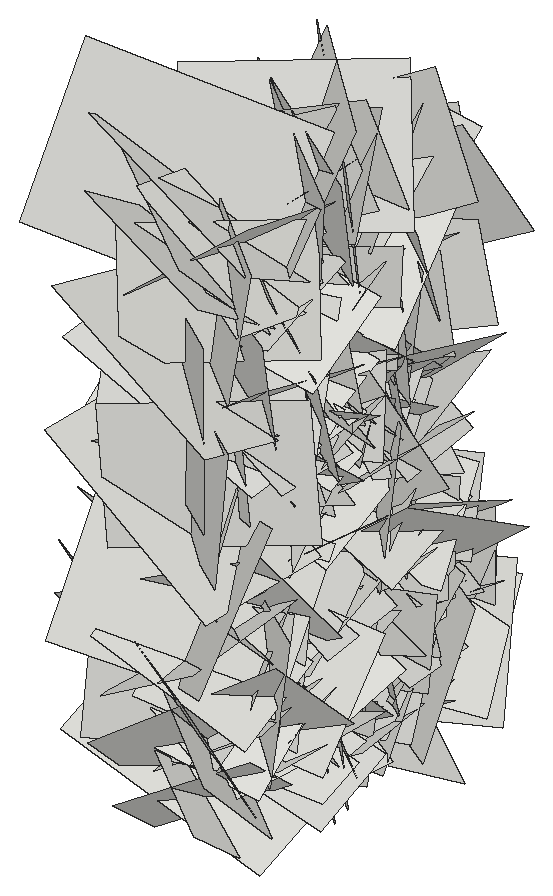
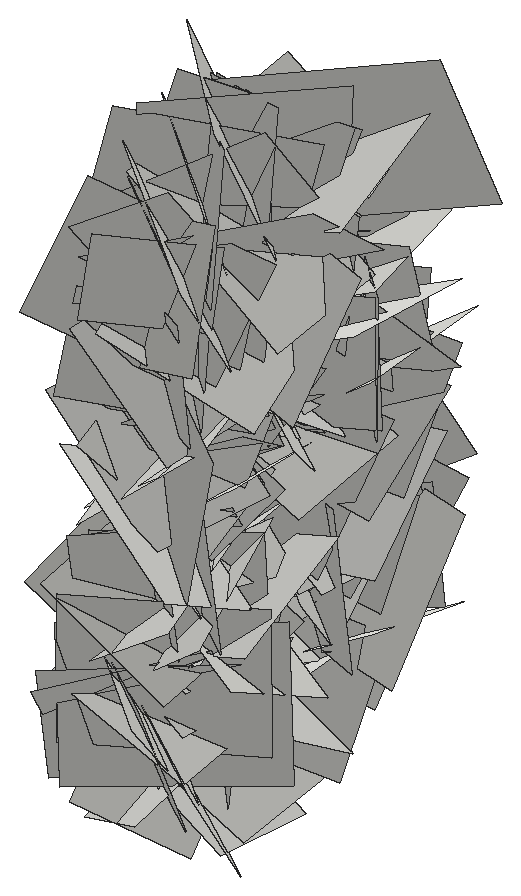
# SketchUp Ruby script. Lengths in inches.
U = 1.inch
M = Sketchup.active_model
def pt(a) = Geom::Point3d.new(a.map { |v| v * U })
def face(e, loops, mat)
  f = e.add_face(loops[0].map { |a| pt(a) })
  loops[1..].each { |l| e.add_face(l.map { |a| pt(a) }).erase! }
  f.material = f.back_material = mat if mat
  f
end
# faces: each face lists its corners as indices into pts; further lists are holes
def faces(e, pts, list, mat = nil) = list.each { |f| face(e, (f[0].is_a?(Array) ? f : [f]).map { |l| l.map { |i| pts[i] } }, mat) }
# xy, xz, yz: faces in a plane at the given z, y or x. An outline is a flat list of corners, or four numbers for a rectangle; further outlines are holes
def ring(l) = l.size == 4 ? [[l[0], l[1]], [l[2], l[1]], [l[2], l[3]], [l[0], l[3]]] : l.each_slice(2).to_a
def flat(e, list, mat, &to3) = list.each { |f| face(e, (f[0].is_a?(Array) ? f : [f]).map { |l| ring(l).map { |u, v| to3.(u, v) } }, mat) }
def xy(e, z, list, mat = nil) = flat(e, list, mat) { |x, y| [x, y, z] }
def xz(e, y, list, mat = nil) = flat(e, list, mat) { |x, z| [x, y, z] }
def yz(e, x, list, mat = nil) = flat(e, list, mat) { |y, z| [x, y, z] }
def lines(e, pts, list) = list.each { |a, b| e.add_line(pt(pts[a]), pt(pts[b])) }
# prism: a flat outline (further loops are holes) pulled along v
def prism(e, loops, v, mat = nil)
  f = face(e, loops, mat); d = Geom::Vector3d.new(v.map { |x| x * U })
  f.pushpull(f.normal.samedirection?(d) ? d.length : -d.length)
end
def box(e, o, s, mat = nil) = prism(e, [[o, [o[0] + s[0], o[1], o[2]], [o[0] + s[0], o[1] + s[1], o[2]], [o[0], o[1] + s[1], o[2]]]], [0, 0, s[2]], mat)
def at(x, y, z, deg = 0) = Geom::Transformation.translation(pt([x, y, z])) * Geom::Transformation.rotation(ORIGIN, Z_AXIS, deg.degrees)
def axes(o, x, y, z) = Geom::Transformation.new([*x, 0, *y, 0, *z, 0, *pt(o).to_a, 1])
def part(name) = M.definitions.add(name)
# library, detail: a bought-in or finely detailed component or shape, given as its bounding box
def library(name, o, s) = part(name).tap { |d| box(d.entities, o, s) }
def detail(e, o, s) = box(e.add_group.entities, o, s)
def put(e, d, t, mat = nil) = e.add_instance(d, t).tap { |i| i.material = mat if mat }
def group(e, t, mat = nil) = e.add_group.tap { |g| g.transformation = t; g.material = mat if mat }.entities
root = M.entities
c1 = part("Component\#6")
p = [[0.01,0,0],[0,3.24,4.54],[4.32,3.24,4.54],[4.33,0,0]]
faces(c1.entities,p,[[0,1,2,3]])
put(root,c1,axes([18.5,141.18,23.91],[-0.20239,-0.45291,-1.29893],[-0.24414,-1.28235,0.48098],[-1.43758,0.28153,0.10118]))
put(root,c1,axes([18.5,137.06,3.09],[-0.11239,-0.69918,1.17187],[-0.18512,1.17269,0.68387],[-1.43458,-0.09655,-0.18006]))
put(root,c1,axes([18.5,140.96,14.21],[-0.1647,-0.56811,1.02456],[-0.16232,1.03452,0.5504],[-1.23116,-0.0604,-0.20963]))
put(root,c1,axes([18.5,141.32,18.93],[0.00931,-1.12138,0.55372],[-0.26786,0.54072,1.09906],[-1.29833,-0.1196,-0.22278]))
put(root,c1,axes([18.5,142.16,14.375],[0.02255,-1.26636,-0.09652],[-0.2141,-0.09868,1.25016],[-1.3291,-0.00559,-0.20302]))
put(root,c1,axes([18.5,139.3125,6.46],[0.05297,-0.89114,0.82127],[-0.332,0.78454,0.87035],[-1.24093,-0.24794,-0.1978]))
put(root,c1,axes([18.5,148.13,7.79],[-0.13698,0.11741,-1.23467],[0.05668,-1.23967,-0.12348],[-1.31343,-0.06574,0.12344]))
put(root,c1,axes([18.5,134.59,13.6],[-0.14779,0.17555,1.29716],[0.16453,1.29751,-0.15892],[-1.37773,0.13612,-0.15813]))
put(root,c1,axes([18.5,141.11,14.91],[-0.10517,-0.78429,-0.79452],[-0.18451,-0.77703,0.78876],[-1.16892,0.19321,-0.05302]))
put(root,c1,axes([18.5,144.73,5.33],[-0.04426,-1.02294,0.56209],[-0.16257,0.56238,1.01208],[-1.2265,-0.03763,-0.15444]))
put(root,c1,axes([18.5,144.3,10.94],[-0.16969,-0.07735,1.18237],[0.06112,1.19119,0.08573],[-1.2545,0.0685,-0.15576]))
put(root,c1,axes([18.5,148.05,8.79],[-0.07068,0.0827,-1.14811],[-0.1221,-1.14474,-0.07576],[-1.21402,0.11031,0.07447]))
put(root,c1,axes([18.5,138.37,16.22],[-0.07456,0.76169,-0.90937],[-0.0504,-0.91204,-0.76025],[-1.25638,-0.00862,0.08446]))
put(root,c1,axes([18.5,141.48,7.17],[-0.20337,0.82379,-0.77749],[0.08888,-0.77608,-0.84298],[-1.19742,-0.19752,0.06948]))
put(root,c1,axes([18.5,139.44,14.86],[0.04621,-1.16691,0.31838],[-0.12643,0.31289,1.16311],[-1.27589,-0.07327,-0.10372]))
put(root,c1,axes([18.5,139.77,22.87],[-0.12093,1.26112,-0.05281],[0.18505,-0.03675,-1.25475],[-1.32509,-0.12022,-0.17041]))
put(root,c1,axes([18.5,146.96,20.2],[0.19126,-1.0536,-0.82739],[-0.10265,-0.84293,1.05228],[-1.41631,-0.08119,-0.188]))
put(root,c1,axes([18.5,137.94,15.45],[0.03401,0.89045,-0.73196],[-0.17038,-0.72163,-0.88493],[-1.2099,0.12665,0.10405]))
put(root,c1,axes([18.5,140.59,7.56],[0.03383,1.06332,0.50099],[-0.10932,0.50178,-1.05842],[-1.24115,-0.01522,0.10688]))
put(root,c1,axes([18.5,140.04,10.48],[0.03722,-1.27767,0.05021],[0.04996,0.05148,1.27723],[-1.35446,-0.03321,0.04849]))
put(root,c1,axes([18.5,143.08,17.68],[0.06532,-0.13436,-1.17102],[-0.13166,-1.16683,0.12734],[-1.24247,0.11658,-0.07506]))
put(root,c1,axes([18.5,141.75,2.91],[0.11729,-1.19784,-0.30033],[-0.11289,-0.30967,1.19584],[-1.30414,-0.08092,-0.13053]))
put(root,c1,axes([18.5,140.93,18.6875],[0.10901,-0.41314,-1.06231],[-0.28274,-1.04573,0.38087],[-1.17466,0.21337,-0.19026]))
put(root,c1,axes([18.5,137.64,18.89],[-0.26376,-0.64139,0.69016],[-0.02251,0.71746,0.65911],[-0.99845,0.15326,-0.19718]))
put(root,c1,axes([18.5,142.88,1.98],[-0.0351,0.64216,0.95117],[-0.00533,0.95147,-0.64254],[-1.21649,-0.02269,-0.02463]))
put(root,c1,axes([18.5,143.17,19.13],[-0.20193,0.9279,-0.28366],[-0.04691,-0.29708,-0.94209],[-1.02744,-0.16881,0.09877]))
put(root,c1,axes([18.5,137.21,11.6875],[0.11385,0.72886,-0.88593],[-0.14818,-0.87485,-0.7367],[-1.20699,0.17615,0.00688]))
put(root,c1,axes([14.53,137.29,3.46],[-0.14224,0.61257,0.15159],[0.04066,0.16261,-0.62315],[0.66768,0.1206,0.07024]))
put(root,c1,axes([18.5,138.49,4.97],[0.13436,1.04009,0.6085],[-0.04809,0.61554,-1.04268],[-1.27641,0.08629,0.10334]))
put(root,c1,axes([18.5,138.64,15.1],[0.05154,1.07135,-0.23626],[-0.10153,-0.23144,-1.06922],[-1.15847,0.06794,0.08319]))
put(root,c1,axes([18.5,142.72,8.07],[0.13823,0.05764,1.30603],[0.0986,1.30878,-0.06705],[-1.38223,0.09912,0.12583]))
put(root,c1,axes([14.53,142.82,6.12],[0.04161,-0.60559,-0.03198],[-0.13563,-0.03959,0.59276],[0.62835,0.03156,0.13006]))
put(root,c1,axes([18.5,143.54,11.83],[0.01207,0.98557,0.48784],[-0.03058,0.48797,-0.98515],[-1.16528,-0.0026,0.03091]))
put(root,c1,axes([18.5,141.07,4.77],[0.0925,1.07709,-0.24358],[-0.13853,-0.23255,-1.07513],[-1.16232,0.11343,0.10875]))
put(root,c1,axes([18.5,137.41,10.49],[-0.17918,0.96529,0.20208],[0.06958,0.21558,-0.97489],[-1.04307,-0.15144,-0.09975]))
put(root,c1,axes([18.5,139.52,8.83],[-0.01584,-0.12995,-1.07448],[-0.00128,-1.07458,0.12998],[-1.14724,0.003,0.01469]))
put(root,c1,axes([18.5,138.76,9.15],[-0.08107,-0.07376,-0.93469],[-0.12107,-0.93007,0.08274],[-0.98644,0.12021,0.06666]))
put(root,c1,axes([18.5,138.34,13.4],[-0.1901,0.66514,0.65147],[0.02496,0.66648,-0.67398],[-0.98658,-0.1113,-0.14258]))
put(root,c1,axes([18.5,141.92,3.18],[-0.02887,1.0089,0.10446],[-0.06921,0.10254,-1.00735],[-1.07292,-0.03376,0.06217]))
put(root,c1,axes([14.53,139.18,13.74],[-0.11062,-0.13563,-0.63299],[0.03095,-0.6415,0.13263],[0.6855,0.00708,-0.10814]))
put(root,c1,axes([18.5,137.89,18.97],[-0.02244,-0.79516,0.48934],[-0.22215,0.48102,0.77258],[-0.96443,-0.0923,-0.18934]))
put(root,c1,axes([18.5,137.63,3.85],[0.23328,-0.07655,1.22947],[-0.08564,1.24535,0.092],[-1.30295,-0.09556,0.21407]))
put(root,c1,axes([14.53,141.95,12.73],[-0.09992,0.55515,0.3498],[0.02862,0.35638,-0.5583],[0.69495,0.06514,0.07329]))
put(root,c1,axes([18.5,146.45,10.34],[-0.10559,0.05407,-0.92917],[-0.0532,-0.93343,-0.04894],[-0.98516,0.04461,0.10223]))
put(root,c1,axes([14.53,145.42,18.19],[-0.07853,-0.05807,0.70782],[-0.06912,0.70921,0.05136],[0.74963,0.05931,0.07889]))
put(root,c1,axes([14.53,145.36,10.15],[-0.14636,-0.64891,0.3527],[-0.01811,0.36152,0.65845],[0.78267,-0.11298,0.08119]))
put(root,c1,axes([14.53,142.6,14.22],[-0.18899,-0.6396,-0.42028],[0.00285,-0.43205,0.65638],[0.81124,-0.14749,-0.10022]))
put(root,c1,axes([14.53,139.8125,20.98],[0.02151,0.52563,-0.34386],[-0.05265,-0.34162,-0.52514],[0.66372,-0.04413,-0.03051]))
put(root,c1,axes([18.5,144.58,9.97],[-0.16827,0.58944,-0.69808],[0.0398,-0.70373,-0.60275],[-0.96765,-0.13145,0.0966]))
put(root,c1,axes([18.5,142.29,19.52],[-0.02505,0.60517,0.90894],[0.1077,0.90642,-0.60085],[-1.15246,0.07156,-0.07591]))
put(root,c1,axes([18.5,137.99,14.66],[0.08461,-0.27233,0.9902],[-0.1352,0.98287,0.28059],[-1.08015,-0.14435,0.04245]))
put(root,c1,axes([18.5,144.34,6.82],[0.01542,0.93301,-0.17325],[-0.14993,-0.1692,-0.92309],[-0.99466,0.03997,0.13646]))
put(root,c1,axes([18.5,141.25,1.55],[-0.11713,-0.0063,1.0149],[0.13715,1.01248,0.02037],[-1.06704,0.13083,-0.10878]))
put(root,c1,axes([18.5,142.2,15.72],[0.2001,0.61396,-1.10583],[0.10306,-1.12181,-0.60624],[-1.33676,0.00542,-0.21228]))
put(root,c1,axes([14.53,138.3,10.21],[-0.07821,-0.14386,0.79141],[-0.12147,0.78851,0.13265],[0.84394,0.10016,0.09244]))
put(root,c1,axes([14.53,147.58,14.43],[-0.15626,-0.88067,0.15465],[-0.14549,0.17716,0.87807],[0.93656,-0.11942,0.1622]))
put(root,c1,axes([14.53,139.99,14.29],[0.01199,-0.16574,0.68191],[-0.09091,0.67656,0.16586],[0.73829,0.086,0.00935]))
put(root,c1,axes([18.5,139.9,15.42],[-0.08068,-0.00169,-0.87701],[-0.08263,-0.87681,0.00845],[-0.92595,0.07839,0.07566]))
put(root,c1,axes([14.53,145.32,5.58],[0.01721,-0.24816,-0.73855],[-0.187,-0.7207,0.23828],[0.80443,-0.16223,0.07119]))
put(root,c1,axes([18.5,140.66,10.67],[0.05387,-0.70807,-1.02445],[0.25854,-0.99979,0.70312],[-1.29449,-0.22915,0.09779]))
put(root,c1,axes([18.5,141.11,17.69],[-0.01651,0.23078,-0.87547],[-0.12637,-0.8685,-0.22682],[-0.95135,0.11136,0.04532]))
put(root,c1,axes([14.53,138.56,10.4375],[-0.05239,0.37979,0.51244],[0.10197,0.51253,-0.37059],[0.66837,-0.04842,0.0967]))
put(root,c1,axes([18.5,149.05,6.52],[0.16475,-0.3536,-1.09271],[0.00842,-1.10231,0.35784],[-1.21738,-0.05548,-0.1454]))
put(root,c1,axes([18.5,142.09,4.39],[-0.13266,-0.06807,0.83796],[-0.05074,0.84639,0.06161],[-0.88972,-0.03812,-0.12846]))
put(root,c1,axes([18.5,136.25,6.15],[-0.02753,0.62765,0.83331],[0.11118,0.83092,-0.62258],[-1.10023,0.06826,-0.08377]))
put(root,c1,axes([14.53,141.82,12.65],[0.04235,0.31596,0.66399],[-0.14644,0.65635,-0.30401],[0.76557,0.10807,-0.09488]))
put(root,c1,axes([18.5,145.41,21.68],[-0.17174,-0.50133,-0.77339],[0.12403,-0.79008,0.48764],[-0.96905,-0.01227,0.19948]))
put(root,c1,axes([14.53,139.97,19.34],[-0.20036,-0.21311,0.82685],[-0.01235,0.84743,0.21575],[0.90502,-0.03562,0.186]))
put(root,c1,axes([18.5,135.11,11.54],[0.10699,0.00448,1.06975],[-0.01257,1.07444,-0.00338],[-1.13388,-0.01149,0.10098]))
put(root,c1,axes([14.53,141.75,2.2],[0.07408,-0.19814,0.56205],[0.01701,0.56632,0.19765],[0.63148,0.00798,-0.07126]))
put(root,c1,axes([18.5,137.79,2.1],[0.03475,-0.78477,0.75119],[0.11687,0.75006,0.77877],[-1.14558,0.05272,0.10224]))
put(root,c1,axes([14.53,139.2,5.38],[-0.02645,-0.5119,-0.36479],[0.13209,-0.36186,0.49927],[0.65307,0.05245,-0.11575]))
put(root,c1,axes([14.53,147.44,21.48],[0.11936,-0.32986,-0.48912],[-0.02265,-0.49991,0.33221],[0.62494,0.04489,0.10546]))
put(root,c1,axes([18.5,139.48,6.78],[-0.1397,0.74364,0.31774],[-0.04551,0.31504,-0.75514],[-0.85599,-0.13812,-0.01171]))
put(root,c1,axes([18.5,146.4375,4.35],[0.18242,-1.06895,0.55133],[0.10581,0.56772,1.06956],[-1.27052,-0.1062,0.16823]))
put(root,c1,axes([14.53,141.96,13.08],[0.07799,-0.57044,-0.33182],[-0.05167,-0.33766,0.56968],[0.69762,0.03877,0.07929]))
put(root,c1,axes([18.5,137.55,18.4],[0.05522,0.7917,0.38208],[-0.20111,0.38385,-0.76951],[-0.90986,-0.0368,0.19328]))
put(root,c1,axes([14.53,140.67,1.375],[0.09858,-0.02009,0.69473],[-0.09996,0.69407,0.03269],[0.72991,0.09776,-0.08935]))
put(root,c1,axes([14.53,143.63,3.63],[0.04495,-0.13338,0.65571],[0.00407,0.65706,0.13341],[0.70927,0.00468,-0.04233]))
put(root,c1,axes([14.53,139.35,17.19],[0.06054,-0.33637,0.61942],[-0.0607,0.61718,0.34043],[0.74468,0.07766,-0.02261]))
put(root,c1,axes([18.5,145.52,15.88],[0.20612,-0.51117,0.96001],[-0.04532,0.97089,0.52562],[-1.15198,-0.12966,0.1511]))
put(root,c1,axes([14.53,136.74,12.93],[0.11437,0.04247,0.59628],[0.02624,0.60507,-0.04758],[0.63311,-0.03275,-0.10574]))
put(root,c1,axes([14.53,142.73,15.75],[-0.26089,1.021,-0.12695],[-0.10549,-0.15355,-1.04195],[1.08548,0.23047,-0.13178]))
put(root,c1,axes([18.5,139.41,15.5],[-0.07329,-0.02436,0.98546],[0.16551,0.97513,0.03506],[-1.03171,0.15816,-0.06438]))
put(root,c1,axes([14.53,143.53,7.33],[-0.11895,-0.88372,0.009],[-0.0734,0.01784,0.88799],[0.93392,-0.11115,0.07094]))
put(root,c1,axes([18.5,142.07,24.73],[0.13514,0.30002,-0.93652],[-0.09595,-0.93677,-0.31242],[-1.03799,0.12565,-0.09305]))
put(root,c1,axes([14.53,138.58,20.36],[-0.30182,0.3301,1.08442],[-0.18064,1.09293,-0.37743],[1.1879,0.25007,0.21813]))
put(root,c1,axes([18.5,143.76,15.19],[-0.09057,0.86782,-0.29614],[0.1091,-0.28647,-0.86917],[-0.96584,-0.11373,-0.07041]))
put(root,c1,axes([18.5,139.77,3.95],[-0.11908,-0.78329,-0.0515],[-0.03618,-0.0471,0.79084],[-0.83129,0.11425,-0.02704]))
put(root,c1,axes([14.53,146.8125,4.55],[-0.17148,-0.83232,0.10491],[0.08015,0.09194,0.84603],[0.88562,-0.16948,-0.05625]))
put(root,c1,axes([18.5,145.52,18.22],[0.02537,0.1253,-0.85934],[-0.08829,-0.85537,-0.12704],[-0.91628,0.08589,-0.01155]))
put(root,c1,axes([18.5,143.66,16.18],[-0.1105,0.58717,-0.52568],[-0.01323,-0.53143,-0.59111],[-0.83529,-0.06926,0.0789]))
put(root,c1,axes([18.5,147.01,9.44],[0.18802,-1.10018,-0.17062],[0.06994,-0.16208,1.11371],[-1.17806,-0.18521,0.03889]))
put(root,c1,axes([14.53,143.33,2.25],[0.06381,-0.71847,0.0034],[-0.02834,0.00117,0.7205],[0.76106,0.06028,0.02655]))
put(root,c1,axes([18.5,144.05,16.5],[-0.02895,-0.76847,-0.41691],[0.01722,-0.41749,0.76847],[-0.92657,0.01625,0.02731]))
put(root,c1,axes([18.5,143.95,11.7],[0.02215,-0.88691,-0.38082],[0.08723,-0.37788,0.88459],[-1.0194,-0.05161,0.06742]))
put(root,c1,axes([14.53,147.56,10.64],[0.00206,-0.13591,-0.77504],[-0.03252,-0.77447,0.13573],[0.83344,-0.02988,0.00721]))
put(root,c1,axes([14.53,142.57,12.97],[-0.12959,-0.66136,0.5647],[0.03976,0.56572,0.67067],[0.92097,-0.11748,0.0505]))
put(root,c1,axes([18.5,141.85,18.04],[0.12661,-0.3078,1.12748],[0.24587,1.11705,0.28038],[-1.21422,0.1941,0.17434]))
put(root,c1,axes([14.53,147.06,19.23],[-0.16196,0.05609,-0.92604],[0.00217,-0.93849,-0.05718],[0.9834,0.01131,-0.15239]))
put(root,c1,axes([14.53,141.5625,11.54],[-0.13399,-0.80117,0.38482],[0.02481,0.38556,0.81039],[0.9418,-0.12414,0.0334]))
put(root,c1,axes([14.53,149.3125,5.88],[-0.15882,-0.57412,-0.80425],[-0.08368,-0.80389,0.58857],[1.04409,-0.15176,-0.07517]))
put(root,c1,axes([18.5,143.03,2.65],[0.18528,-0.93043,-0.12384],[-0.14778,-0.15031,0.9325],[-0.98392,-0.15263,-0.16338]))
put(root,c1,axes([14.53,141.35,5.69],[0.05421,0.52298,-0.48745],[0.04158,-0.49001,-0.52162],[0.75668,-0.01054,0.06359]))
put(root,c1,axes([18.5,145.65,3.28],[-0.1646,0.60158,-0.34623],[-0.0091,-0.35642,-0.61544],[-0.73568,-0.13018,0.08507]))
put(root,c1,axes([14.53,139.62,7.21],[-0.15609,-0.9187,-0.23757],[-0.00588,-0.23958,0.92989],[1.00583,-0.14396,-0.03143]))
put(root,c1,axes([14.53,143.17,8.1],[0.04482,0.75985,0.07181],[0.00358,0.07173,-0.76102],[0.80902,-0.04241,-0.00061]))
put(root,c1,axes([14.53,141.47,13.3125],[-0.15098,-0.93805,0.13539],[-0.00567,0.13771,0.94846],[1.00463,-0.1402,0.0257]))
put(root,c1,axes([18.5,139.94,18.75],[0.02341,-0.9115,0.17831],[0.09444,0.17962,0.90714],[-0.97996,-0.00447,0.09169]))
put(root,c1,axes([14.53,144.39,10.35],[-0.12238,0.87118,-0.30871],[-0.00416,-0.31157,-0.87778],[0.97971,0.1075,-0.04229]))
put(root,c1,axes([14.53,135.6875,17.375],[-0.11773,0.10526,0.9962],[-0.108,0.99592,-0.11659],[1.05635,0.11356,0.09911]))
put(root,c1,axes([14.53,136.7,5.12],[0.11008,0.58852,-0.4619],[-0.03608,-0.46213,-0.59646],[0.7922,-0.10282,0.03702]))
put(root,c1,axes([18.5,147.32,10.4375],[0.06119,-0.47987,-0.75245],[0.01649,-0.75336,0.48165],[-0.94584,-0.04418,-0.04028]))
put(root,c1,axes([14.53,147.32,10.4375],[-0.06119,-0.47987,-0.75245],[-0.01649,-0.75336,0.48165],[0.94584,-0.04418,-0.04028]))
put(root,c1,axes([18.5,136.7,5.12],[-0.11008,0.58852,-0.4619],[0.03608,-0.46213,-0.59646],[-0.7922,-0.10282,0.03702]))
put(root,c1,axes([18.5,135.6875,17.375],[0.11773,0.10526,0.9962],[0.108,0.99592,-0.11659],[-1.05635,0.11356,0.09911]))
put(root,c1,axes([18.5,144.39,10.35],[0.12238,0.87118,-0.30871],[0.00416,-0.31157,-0.87778],[-0.97971,0.1075,-0.04229]))
put(root,c1,axes([14.53,139.94,18.75],[-0.02341,-0.9115,0.17831],[-0.09444,0.17962,0.90714],[0.97996,-0.00447,0.09169]))
put(root,c1,axes([18.5,141.47,13.3125],[0.15098,-0.93805,0.13539],[0.00567,0.13771,0.94846],[-1.00463,-0.1402,0.0257]))
put(root,c1,axes([18.5,143.17,8.1],[-0.04482,0.75985,0.07181],[-0.00358,0.07173,-0.76102],[-0.80902,-0.04241,-0.00061]))
put(root,c1,axes([18.5,139.62,7.21],[0.15609,-0.9187,-0.23757],[0.00588,-0.23958,0.92989],[-1.00583,-0.14396,-0.03143]))
put(root,c1,axes([14.53,145.65,3.28],[0.1646,0.60158,-0.34623],[0.0091,-0.35642,-0.61544],[0.73568,-0.13018,0.08507]))
put(root,c1,axes([18.5,141.35,5.69],[-0.05421,0.52298,-0.48745],[-0.04158,-0.49001,-0.52162],[-0.75668,-0.01054,0.06359]))
put(root,c1,axes([14.53,143.03,2.65],[-0.18528,-0.93043,-0.12384],[0.14778,-0.15031,0.9325],[0.98392,-0.15263,-0.16338]))
put(root,c1,axes([18.5,149.3125,5.88],[0.15882,-0.57412,-0.80425],[0.08368,-0.80389,0.58857],[-1.04409,-0.15176,-0.07517]))
put(root,c1,axes([18.5,141.5625,11.54],[0.13399,-0.80117,0.38482],[-0.02481,0.38556,0.81039],[-0.9418,-0.12414,0.0334]))
put(root,c1,axes([18.5,147.06,19.23],[0.16196,0.05609,-0.92604],[-0.00217,-0.93849,-0.05718],[-0.9834,0.01131,-0.15239]))
put(root,c1,axes([14.53,141.85,18.04],[-0.12661,-0.3078,1.12748],[-0.24587,1.11705,0.28038],[1.21422,0.1941,0.17434]))
put(root,c1,axes([18.5,142.57,12.97],[0.12959,-0.66136,0.5647],[-0.03976,0.56572,0.67067],[-0.92097,-0.11748,0.0505]))
put(root,c1,axes([18.5,147.56,10.64],[-0.00206,-0.13591,-0.77504],[0.03252,-0.77447,0.13573],[-0.83344,-0.02988,0.00721]))
put(root,c1,axes([14.53,143.95,11.7],[-0.02215,-0.88691,-0.38082],[-0.08723,-0.37788,0.88459],[1.0194,-0.05161,0.06742]))
put(root,c1,axes([14.53,144.05,16.5],[0.02895,-0.76847,-0.41691],[-0.01722,-0.41749,0.76847],[0.92657,0.01625,0.02731]))
put(root,c1,axes([18.5,143.33,2.25],[-0.06381,-0.71847,0.0034],[0.02834,0.00117,0.7205],[-0.76106,0.06028,0.02655]))
put(root,c1,axes([14.53,147.01,9.44],[-0.18802,-1.10018,-0.17062],[-0.06994,-0.16208,1.11371],[1.17806,-0.18521,0.03889]))
put(root,c1,axes([14.53,143.66,16.18],[0.1105,0.58717,-0.52568],[0.01323,-0.53143,-0.59111],[0.83529,-0.06926,0.0789]))
put(root,c1,axes([14.53,145.52,18.22],[-0.02537,0.1253,-0.85934],[0.08829,-0.85537,-0.12704],[0.91628,0.08589,-0.01155]))
put(root,c1,axes([18.5,146.8125,4.55],[0.17148,-0.83232,0.10491],[-0.08015,0.09194,0.84603],[-0.88562,-0.16948,-0.05625]))
put(root,c1,axes([14.53,139.77,3.95],[0.11908,-0.78329,-0.0515],[0.03618,-0.0471,0.79084],[0.83129,0.11425,-0.02704]))
put(root,c1,axes([14.53,143.76,15.19],[0.09057,0.86782,-0.29614],[-0.1091,-0.28647,-0.86917],[0.96584,-0.11373,-0.07041]))
put(root,c1,axes([18.5,138.58,20.36],[0.30182,0.3301,1.08442],[0.18064,1.09293,-0.37743],[-1.1879,0.25007,0.21813]))
put(root,c1,axes([14.53,142.07,24.73],[-0.13514,0.30002,-0.93652],[0.09595,-0.93677,-0.31242],[1.03799,0.12565,-0.09305]))
put(root,c1,axes([18.5,143.53,7.33],[0.11895,-0.88372,0.009],[0.0734,0.01784,0.88799],[-0.93392,-0.11115,0.07094]))
put(root,c1,axes([14.53,139.41,15.5],[0.07329,-0.02436,0.98546],[-0.16551,0.97513,0.03506],[1.03171,0.15816,-0.06438]))
put(root,c1,axes([18.5,142.73,15.75],[0.26089,1.021,-0.12695],[0.10549,-0.15355,-1.04195],[-1.08548,0.23047,-0.13178]))
put(root,c1,axes([18.5,136.74,12.93],[-0.11437,0.04247,0.59628],[-0.02624,0.60507,-0.04758],[-0.63311,-0.03275,-0.10574]))
put(root,c1,axes([14.53,145.52,15.88],[-0.20612,-0.51117,0.96001],[0.04532,0.97089,0.52562],[1.15198,-0.12966,0.1511]))
put(root,c1,axes([18.5,139.35,17.19],[-0.06054,-0.33637,0.61942],[0.0607,0.61718,0.34043],[-0.74468,0.07766,-0.02261]))
put(root,c1,axes([18.5,143.63,3.63],[-0.04495,-0.13338,0.65571],[-0.00407,0.65706,0.13341],[-0.70927,0.00468,-0.04233]))
put(root,c1,axes([18.5,140.67,1.375],[-0.09858,-0.02009,0.69473],[0.09996,0.69407,0.03269],[-0.72991,0.09776,-0.08935]))
put(root,c1,axes([14.53,137.55,18.4],[-0.05522,0.7917,0.38208],[0.20111,0.38385,-0.76951],[0.90986,-0.0368,0.19328]))
put(root,c1,axes([18.5,141.96,13.08],[-0.07799,-0.57044,-0.33182],[0.05167,-0.33766,0.56968],[-0.69762,0.03877,0.07929]))
put(root,c1,axes([14.53,146.4375,4.35],[-0.18242,-1.06895,0.55133],[-0.10581,0.56772,1.06956],[1.27052,-0.1062,0.16823]))
put(root,c1,axes([14.53,139.48,6.78],[0.1397,0.74364,0.31774],[0.04551,0.31504,-0.75514],[0.85599,-0.13812,-0.01171]))
put(root,c1,axes([18.5,147.44,21.48],[-0.11936,-0.32986,-0.48912],[0.02265,-0.49991,0.33221],[-0.62494,0.04489,0.10546]))
put(root,c1,axes([18.5,139.2,5.38],[0.02645,-0.5119,-0.36479],[-0.13209,-0.36186,0.49927],[-0.65307,0.05245,-0.11575]))
put(root,c1,axes([14.53,137.79,2.1],[-0.03475,-0.78477,0.75119],[-0.11687,0.75006,0.77877],[1.14558,0.05272,0.10224]))
put(root,c1,axes([18.5,141.75,2.2],[-0.07408,-0.19814,0.56205],[-0.01701,0.56632,0.19765],[-0.63148,0.00798,-0.07126]))
put(root,c1,axes([14.53,135.11,11.54],[-0.10699,0.00448,1.06975],[0.01257,1.07444,-0.00338],[1.13388,-0.01149,0.10098]))
put(root,c1,axes([18.5,139.97,19.34],[0.20036,-0.21311,0.82685],[0.01235,0.84743,0.21575],[-0.90502,-0.03562,0.186]))
put(root,c1,axes([14.53,145.41,21.68],[0.17174,-0.50133,-0.77339],[-0.12403,-0.79008,0.48764],[0.96905,-0.01227,0.19948]))
put(root,c1,axes([18.5,141.82,12.65],[-0.04235,0.31596,0.66399],[0.14644,0.65635,-0.30401],[-0.76557,0.10807,-0.09488]))
put(root,c1,axes([14.53,136.25,6.15],[0.02753,0.62765,0.83331],[-0.11118,0.83092,-0.62258],[1.10023,0.06826,-0.08377]))
put(root,c1,axes([14.53,142.09,4.39],[0.13266,-0.06807,0.83796],[0.05074,0.84639,0.06161],[0.88972,-0.03812,-0.12846]))
put(root,c1,axes([14.53,149.05,6.52],[-0.16475,-0.3536,-1.09271],[-0.00842,-1.10231,0.35784],[1.21738,-0.05548,-0.1454]))
put(root,c1,axes([18.5,138.56,10.4375],[0.05239,0.37979,0.51244],[-0.10197,0.51253,-0.37059],[-0.66837,-0.04842,0.0967]))
put(root,c1,axes([14.53,141.11,17.69],[0.01651,0.23078,-0.87547],[0.12637,-0.8685,-0.22682],[0.95135,0.11136,0.04532]))
put(root,c1,axes([14.53,140.66,10.67],[-0.05387,-0.70807,-1.02445],[-0.25854,-0.99979,0.70312],[1.29449,-0.22915,0.09779]))
put(root,c1,axes([18.5,145.32,5.58],[-0.01721,-0.24816,-0.73855],[0.187,-0.7207,0.23828],[-0.80443,-0.16223,0.07119]))
